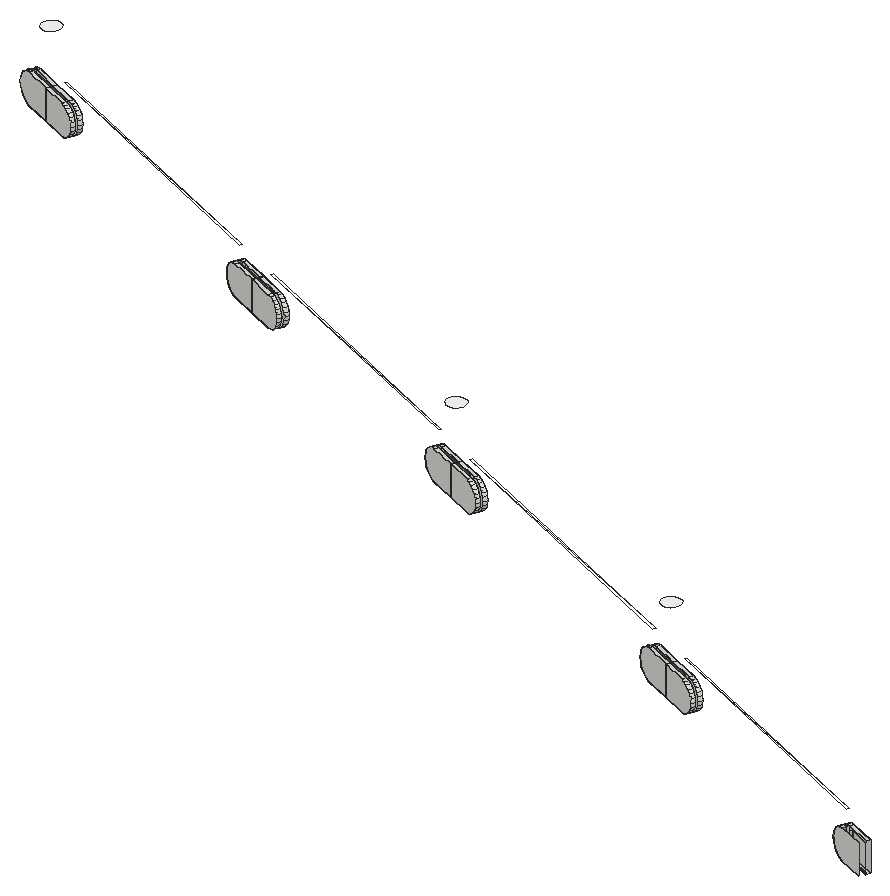
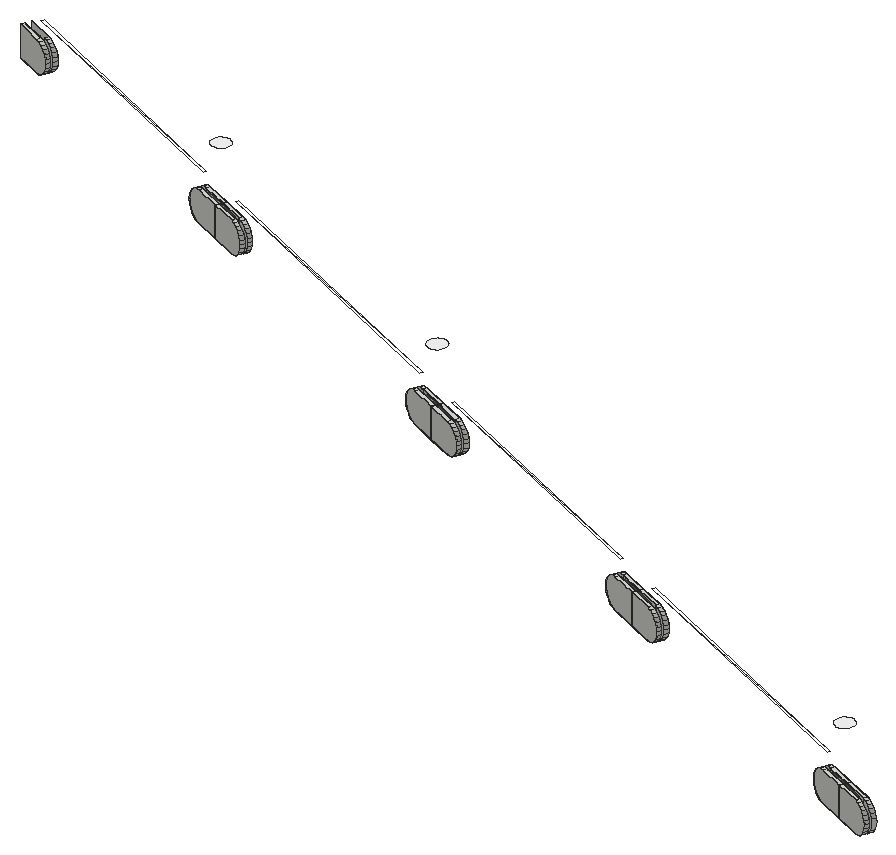
# SketchUp Ruby script. Lengths in inches.
U = 1.inch
M = Sketchup.active_model
def pt(a) = Geom::Point3d.new(a.map { |v| v * U })
def face(e, loops, mat)
  f = e.add_face(loops[0].map { |a| pt(a) })
  loops[1..].each { |l| e.add_face(l.map { |a| pt(a) }).erase! }
  f.material = f.back_material = mat if mat
  f
end
# faces: each face lists its corners as indices into pts; further lists are holes
def faces(e, pts, list, mat = nil) = list.each { |f| face(e, (f[0].is_a?(Array) ? f : [f]).map { |l| l.map { |i| pts[i] } }, mat) }
# xy, xz, yz: faces in a plane at the given z, y or x. An outline is a flat list of corners, or four numbers for a rectangle; further outlines are holes
def ring(l) = l.size == 4 ? [[l[0], l[1]], [l[2], l[1]], [l[2], l[3]], [l[0], l[3]]] : l.each_slice(2).to_a
def flat(e, list, mat, &to3) = list.each { |f| face(e, (f[0].is_a?(Array) ? f : [f]).map { |l| ring(l).map { |u, v| to3.(u, v) } }, mat) }
def xy(e, z, list, mat = nil) = flat(e, list, mat) { |x, y| [x, y, z] }
def xz(e, y, list, mat = nil) = flat(e, list, mat) { |x, z| [x, y, z] }
def yz(e, x, list, mat = nil) = flat(e, list, mat) { |y, z| [x, y, z] }
def lines(e, pts, list) = list.each { |a, b| e.add_line(pt(pts[a]), pt(pts[b])) }
# prism: a flat outline (further loops are holes) pulled along v
def prism(e, loops, v, mat = nil)
  f = face(e, loops, mat); d = Geom::Vector3d.new(v.map { |x| x * U })
  f.pushpull(f.normal.samedirection?(d) ? d.length : -d.length)
end
def box(e, o, s, mat = nil) = prism(e, [[o, [o[0] + s[0], o[1], o[2]], [o[0] + s[0], o[1] + s[1], o[2]], [o[0], o[1] + s[1], o[2]]]], [0, 0, s[2]], mat)
def at(x, y, z, deg = 0) = Geom::Transformation.translation(pt([x, y, z])) * Geom::Transformation.rotation(ORIGIN, Z_AXIS, deg.degrees)
def axes(o, x, y, z) = Geom::Transformation.new([*x, 0, *y, 0, *z, 0, *pt(o).to_a, 1])
def part(name) = M.definitions.add(name)
# library, detail: a bought-in or finely detailed component or shape, given as its bounding box
def library(name, o, s) = part(name).tap { |d| box(d.entities, o, s) }
def detail(e, o, s) = box(e.add_group.entities, o, s)
def put(e, d, t, mat = nil) = e.add_instance(d, t).tap { |i| i.material = mat if mat }
def group(e, t, mat = nil) = e.add_group.tap { |g| g.transformation = t; g.material = mat if mat }.entities
root = M.entities
M.materials.add("Glass_Safety_01").color = [204, 235, 244]
M.materials["Glass_Safety_01"].alpha = 0.1
M.materials.add("[Color_000]").color = [255, 255, 255]
xy(root,351.28,[[937.98,1050.01,936.18,1050.79,936.29,1051.04,938.09,1050.26],[918.36,1058.03,916.56,1058.82,916.67,1059.07,918.32,1058.35,918.47,1058.29],[918.55,1058.47,918.4,1058.53,916.75,1059.25,916.86,1059.51,918.66,1058.72],[916.56,1058.82,914.75,1059.61,914.86,1059.86,916.67,1059.07],[916.75,1059.25,914.94,1060.04,915.05,1060.29,916.86,1059.51],
  [894.73,1068.32,892.93,1069.11,893.04,1069.36,894.71,1068.64,894.84,1068.58],[894.92,1068.76,894.79,1068.82,893.12,1069.54,893.23,1069.8,895.03,1069.01],[892.93,1069.11,891.125,1069.9,891.24,1070.15,893.04,1069.36],[893.12,1069.54,891.3125,1070.33,891.42,1070.58,893.23,1069.8],[872.89,1077.84,871.09,1078.625,871.2,1078.88,872.85,1078.16,873,1078.09],
  [873.08,1078.27,872.93,1078.34,871.27,1079.06,871.38,1079.31,873.19,1078.52],[871.09,1078.625,869.28,1079.41,869.39,1079.66,871.2,1078.88],[871.27,1079.06,869.47,1079.84,869.58,1080.1,871.38,1079.31],[850.22,1087.71,848.42,1088.5,848.53,1088.75,850.19,1088.03,850.33,1087.96],[850.41,1088.14,850.27,1088.21,848.61,1088.93,848.72,1089.18,850.52,1088.4],
  [848.42,1088.5,846.62,1089.28,846.73,1089.54,848.53,1088.75],[848.61,1088.93,846.8,1089.72,846.91,1089.97,848.72,1089.18]])
xy(root,351.36,[[918.11,1058.44,916.67,1059.07,916.75,1059.25,918.19,1058.625],[916.67,1059.07,915.23,1059.7,915.3,1059.88,916.75,1059.25],[894.48,1068.73,893.04,1069.36,893.12,1069.54,894.5625,1068.92],[893.04,1069.36,891.6,1069.99,891.67,1070.17,893.12,1069.54],[872.64,1078.25,871.2,1078.88,871.27,1079.06,872.72,1078.43],
  [871.2,1078.88,869.75,1079.51,869.83,1079.6875,871.27,1079.06],[849.97,1088.12,848.53,1088.75,848.61,1088.93,850.05,1088.3],[848.53,1088.75,847.09,1089.38,847.16,1089.56,848.61,1088.93]],"Glass_Safety_01")
xy(root,353.33,[[918.11,1058.44,918.19,1058.625,916.75,1059.25,916.67,1059.07],[916.67,1059.07,916.75,1059.25,915.3,1059.88,915.23,1059.7],[894.48,1068.73,894.5625,1068.92,893.12,1069.54,893.04,1069.36],[893.04,1069.36,893.12,1069.54,891.67,1070.17,891.6,1069.99],[872.64,1078.25,872.72,1078.43,871.27,1079.06,871.2,1078.88],
  [871.2,1078.88,871.27,1079.06,869.83,1079.6875,869.75,1079.51],[849.97,1088.12,850.05,1088.3,848.61,1088.93,848.53,1088.75],[848.53,1088.75,848.61,1088.93,847.16,1089.56,847.09,1089.38]],"Glass_Safety_01")
xy(root,353.41,[[937.98,1050.01,938.09,1050.26,936.29,1051.04,936.18,1050.79],[918.36,1058.03,918.47,1058.29,918.32,1058.35,916.67,1059.07,916.56,1058.82],[918.55,1058.47,918.66,1058.72,916.86,1059.51,916.75,1059.25,918.4,1058.53],[916.56,1058.82,916.67,1059.07,914.86,1059.86,914.75,1059.61],[916.75,1059.25,916.86,1059.51,915.05,1060.29,914.94,1060.04],
  [894.73,1068.32,894.84,1068.58,894.71,1068.64,893.04,1069.36,892.93,1069.11],[894.92,1068.76,895.03,1069.01,893.23,1069.8,893.12,1069.54,894.79,1068.82],[892.93,1069.11,893.04,1069.36,891.24,1070.15,891.125,1069.9],[893.12,1069.54,893.23,1069.8,891.42,1070.58,891.3125,1070.33],[872.89,1077.84,873,1078.09,872.85,1078.16,871.2,1078.88,871.09,1078.625],
  [873.08,1078.27,873.19,1078.52,871.38,1079.31,871.27,1079.06,872.93,1078.34],[871.09,1078.625,871.2,1078.88,869.39,1079.66,869.28,1079.41],[871.27,1079.06,871.38,1079.31,869.58,1080.1,869.47,1079.84],[850.22,1087.71,850.33,1087.96,850.19,1088.03,848.53,1088.75,848.42,1088.5],[850.41,1088.14,850.52,1088.4,848.72,1089.18,848.61,1088.93,850.27,1088.21],
  [848.42,1088.5,848.53,1088.75,846.73,1089.54,846.62,1089.28],[848.61,1088.93,848.72,1089.18,846.91,1089.97,846.8,1089.72]])
xy(root,354.51,[[936.1,1050.61,936.18,1050.79,918.32,1058.35],[936.18,1050.79,918.4,1058.53,918.32,1058.35],[914.86,1059.86,914.94,1060.04,894.71,1068.64],[914.94,1060.04,894.79,1068.82,894.71,1068.64],[891.24,1070.15,891.3125,1070.33,872.85,1078.16],
  [891.3125,1070.33,872.93,1078.34,872.85,1078.16],[869.39,1079.66,869.47,1079.84,850.19,1088.03],[869.47,1079.84,850.27,1088.21,850.19,1088.03]],"Glass_Safety_01")
xy(root,357.27,[[916.75,1058.53,916.91,1058.57,917.0625,1058.64,917.18,1058.75,917.27,1058.89,917.33,1059.04,917.34,1059.21,917.3,1059.37,917.23,1059.52,917.12,1059.64,916.98,1059.73,916.83,1059.78,916.66,1059.79,916.5,1059.76,916.36,1059.68,916.23,1059.58,916.14,1059.4375,916.09,1059.28,916.08,1059.12,916.11,1058.96,916.1875,1058.81,916.3,1058.6875,916.43,1058.6,916.59,1058.54],[893.125,1068.83,893.29,1068.86,893.43,1068.93,893.56,1069.04,893.65,1069.18,893.7,1069.33,893.71,1069.5,893.67,1069.66,893.6,1069.81,893.49,1069.93,893.35,1070.02,893.2,1070.07,893.03,1070.08,892.875,1070.05,892.73,1069.98,892.6,1069.87,892.51,1069.73,892.46,1069.57,892.45,1069.41,892.48,1069.25,892.56,1069.1,892.67,1068.98,892.8,1068.89,892.96,1068.84],[848.61,1088.21,848.78,1088.24,848.92,1088.32,849.05,1088.43,849.14,1088.5625,849.1875,1088.72,849.2,1088.88,849.16,1089.05,849.09,1089.19,848.98,1089.32,848.84,1089.41,848.6875,1089.46,848.52,1089.47,848.36,1089.43,848.22,1089.36,848.09,1089.25,848,1089.11,847.95,1088.96,847.94,1088.79,847.97,1088.63,848.05,1088.49,848.16,1088.36,848.29,1088.27,848.45,1088.22]],"[Color_000]")
p = [[937.79,1049.57,353.41],[935.99,1050.36,353.41],[935.74,1050.47,353.37],[935.5,1050.57,353.27],[935.3,1050.66,353.1],[935.14,1050.73,352.88],
  [935.05,1050.77,352.62],[935.01,1050.78,352.35],[935.05,1050.77,352.07],[935.14,1050.73,351.8125],[935.3,1050.66,351.59],[935.5,1050.57,351.43],
  [935.74,1050.47,351.32],[935.99,1050.36,351.28],[937.79,1049.57,351.28],[937.98,1050.01,353.41],[936.18,1050.79,353.41],[936.18,1050.79,351.28],
  [937.98,1050.01,351.28],[937.98,1050.01,351.36],[936.54,1050.63,351.36],[936.54,1050.63,353.33],[937.98,1050.01,353.33],[936.29,1051.04,353.41],
  [938.09,1050.26,353.41],[938.09,1050.26,351.28],[936.29,1051.04,351.28],[936.03,1051.15,351.32],[935.8,1051.26,351.43],[935.6,1051.34,351.59],
  [935.44,1051.41,351.8125],[935.34,1051.45,352.07],[935.3125,1051.47,352.35],[935.34,1051.45,352.62],[935.44,1051.41,352.88],[935.6,1051.34,353.1],
  [935.8,1051.26,353.27],[936.03,1051.15,353.37],[935.85,1050.72,351.32],[936.1,1050.61,351.28],[935.61,1050.82,351.43],[936.1,1050.61,353.41],
  [935.85,1050.72,353.37],[935.61,1050.82,353.27],[935.41,1050.91,353.1],[935.25,1050.98,352.88],[935.16,1051.02,352.62],[935.12,1051.04,352.35],
  [935.16,1051.02,352.07],[935.25,1050.98,351.8125],[935.41,1050.91,351.59],[935.92,1050.9,351.32],[935.6875,1051,351.43],[935.49,1051.09,351.59],
  [935.33,1051.16,351.8125],[935.23,1051.2,352.07],[935.2,1051.22,352.35],[935.23,1051.2,352.62],[935.33,1051.16,352.88],[935.49,1051.09,353.1],
  [935.6875,1051,353.27],[935.92,1050.9,353.37],[918.36,1058.03,353.41],[916.56,1058.82,353.41],[916.56,1058.82,351.28],[918.36,1058.03,351.28],
  [918.62,1057.92,351.32],[918.85,1057.82,351.43],[919.05,1057.73,351.59],[919.21,1057.67,351.8125],[919.3,1057.625,352.07],[919.34,1057.61,352.35],
  [919.3,1057.625,352.62],[919.21,1057.67,352.88],[919.05,1057.73,353.1],[918.85,1057.82,353.27],[918.62,1057.92,353.37],[918.73,1058.18,351.32],
  [918.96,1058.07,351.43],[918.47,1058.29,351.28],[918.32,1058.35,351.28],[918.32,1058.35,353.41],[918.47,1058.29,353.41],[918.73,1058.18,353.37],
  [918.96,1058.07,353.27],[919.16,1057.99,353.1],[919.32,1057.92,352.88],[919.42,1057.875,352.62],[919.45,1057.86,352.35],[919.42,1057.875,352.07],
  [919.32,1057.92,351.8125],[919.16,1057.99,351.59],[918.55,1058.47,353.41],[918.4,1058.53,353.41],[918.4,1058.53,351.28],[918.55,1058.47,351.28],
  [918.8,1058.36,351.32],[919.04,1058.25,351.43],[919.24,1058.17,351.59],[919.4,1058.1,351.8125],[919.49,1058.06,352.07],[919.53,1058.04,352.35],
  [919.49,1058.06,352.62],[919.4,1058.1,352.88],[919.24,1058.17,353.1],[919.04,1058.25,353.27],[918.8,1058.36,353.37],[916.86,1059.51,353.41],
  [918.66,1058.72,353.41],[918.91,1058.61,353.37],[919.15,1058.51,353.27],[919.35,1058.42,353.1],[919.51,1058.35,352.88],[919.6,1058.31,352.62],
  [919.64,1058.3,352.35],[919.6,1058.31,352.07],[919.51,1058.35,351.8125],[919.35,1058.42,351.59],[919.15,1058.51,351.43],[918.91,1058.61,351.32],
  [918.66,1058.72,351.28],[916.86,1059.51,351.28],[916.67,1059.07,353.41],[916.67,1059.07,351.28],[916.67,1059.07,351.36],[918.11,1058.44,351.36],
  [918.11,1058.44,353.33],[916.67,1059.07,353.33],[916.75,1059.25,351.28],[916.75,1059.25,353.41],[916.75,1059.25,353.33],[918.19,1058.625,353.33],
  [918.19,1058.625,351.36],[916.75,1059.25,351.36],[914.75,1059.61,353.41],[914.5,1059.72,353.37],[914.27,1059.82,353.27],[914.06,1059.91,353.1],
  [913.91,1059.97,352.88],[913.8125,1060.02,352.62],[913.78,1060.03,352.35],[913.8125,1060.02,352.07],[913.91,1059.97,351.8125],[914.06,1059.91,351.59],
  [914.27,1059.82,351.43],[914.5,1059.72,351.32],[914.75,1059.61,351.28],[914.86,1059.86,351.28],[914.86,1059.86,353.41],[915.23,1059.7,353.33],
  [915.23,1059.7,351.36],[914.94,1060.04,353.41],[914.94,1060.04,351.28],[915.3,1059.88,351.36],[915.3,1059.88,353.33],[915.05,1060.29,353.41],
  [915.05,1060.29,351.28],[914.8,1060.4,351.32],[914.57,1060.5,351.43],[914.36,1060.59,351.59],[914.21,1060.66,351.8125],[914.11,1060.7,352.07],
  [914.08,1060.72,352.35],[914.11,1060.7,352.62],[914.21,1060.66,352.88],[914.36,1060.59,353.1],[914.57,1060.5,353.27],[914.8,1060.4,353.37],
  [914.61,1059.97,351.32],[914.375,1060.07,351.43],[914.61,1059.97,353.37],[914.375,1060.07,353.27],[914.17,1060.16,353.1],[914.02,1060.23,352.88],
  [913.92,1060.27,352.62],[913.89,1060.28,352.35],[913.92,1060.27,352.07],[914.02,1060.23,351.8125],[914.17,1060.16,351.59],[914.69,1060.15,351.32],
  [914.46,1060.25,351.43],[914.25,1060.34,351.59],[914.1,1060.41,351.8125],[914,1060.45,352.07],[913.97,1060.46,352.35],[914,1060.45,352.62],
  [914.1,1060.41,352.88],[914.25,1060.34,353.1],[914.46,1060.25,353.27],[914.69,1060.15,353.37],[894.73,1068.32,353.41],[892.93,1069.11,353.41],
  [892.93,1069.11,351.28],[894.73,1068.32,351.28],[894.99,1068.22,351.32],[895.22,1068.11,351.43],[895.42,1068.02,351.59],[895.58,1067.96,351.8125],
  [895.68,1067.91,352.07],[895.71,1067.9,352.35],[895.68,1067.91,352.62],[895.58,1067.96,352.88],[895.42,1068.02,353.1],[895.22,1068.11,353.27],
  [894.99,1068.22,353.37],[895.1,1068.47,351.32],[895.33,1068.37,351.43],[894.84,1068.58,351.28],[894.71,1068.64,351.28],[894.71,1068.64,353.41],
  [894.84,1068.58,353.41],[895.1,1068.47,353.37],[895.33,1068.37,353.27],[895.53,1068.28,353.1],[895.6875,1068.21,352.88],[895.79,1068.17,352.62],
  [895.82,1068.15,352.35],[895.79,1068.17,352.07],[895.6875,1068.21,351.8125],[895.53,1068.28,351.59],[894.92,1068.76,353.41],[894.79,1068.82,353.41],
  [894.79,1068.82,351.28],[894.92,1068.76,351.28],[895.18,1068.65,351.32],[895.41,1068.55,351.43],[895.61,1068.46,351.59],[895.77,1068.39,351.8125],
  [895.86,1068.35,352.07],[895.9,1068.33,352.35],[895.86,1068.35,352.62],[895.77,1068.39,352.88],[895.61,1068.46,353.1],[895.41,1068.55,353.27],
  [895.18,1068.65,353.37],[895.29,1068.9,351.32],[895.52,1068.8,351.43],[893.04,1069.36,353.41],[893.04,1069.36,351.28],[893.04,1069.36,351.36],
  [894.48,1068.73,351.36],[894.48,1068.73,353.33],[893.04,1069.36,353.33],[893.23,1069.8,353.41],[895.03,1069.01,353.41],[895.29,1068.9,353.37],
  [895.52,1068.8,353.27],[895.72,1068.71,353.1],[895.88,1068.64,352.88],[895.97,1068.6,352.62],[896.01,1068.59,352.35],[895.97,1068.6,352.07],
  [895.88,1068.64,351.8125],[895.72,1068.71,351.59],[895.03,1069.01,351.28],[893.23,1069.8,351.28],[893.12,1069.54,351.28],[893.12,1069.54,353.41],
  [893.12,1069.54,353.33],[894.5625,1068.92,353.33],[894.5625,1068.92,351.36],[893.12,1069.54,351.36],[891.125,1069.9,353.41],[890.87,1070.01,353.37],
  [890.64,1070.11,353.27],[890.4375,1070.2,353.1],[890.28,1070.26,352.88],[890.18,1070.31,352.62],[890.15,1070.32,352.35],[890.18,1070.31,352.07],
  [890.28,1070.26,351.8125],[890.4375,1070.2,351.59],[890.64,1070.11,351.43],[890.87,1070.01,351.32],[891.125,1069.9,351.28],[891.24,1070.15,351.28],
  [891.24,1070.15,353.41],[891.6,1069.99,353.33],[891.6,1069.99,351.36],[891.3125,1070.33,353.41],[891.3125,1070.33,351.28],[891.67,1070.17,351.36],
  [891.67,1070.17,353.33],[891.42,1070.58,353.41],[891.42,1070.58,351.28],[891.17,1070.69,351.32],[890.9375,1070.79,351.43],[890.73,1070.88,351.59],
  [890.58,1070.95,351.8125],[890.48,1070.99,352.07],[890.45,1071.01,352.35],[890.48,1070.99,352.62],[890.58,1070.95,352.88],[890.73,1070.88,353.1],
  [890.9375,1070.79,353.27],[891.17,1070.69,353.37],[890.98,1070.26,351.32],[890.75,1070.36,351.43],[890.98,1070.26,353.37],[890.75,1070.36,353.27],
  [890.55,1070.45,353.1],[890.39,1070.52,352.88],[890.29,1070.56,352.62],[890.26,1070.57,352.35],[890.29,1070.56,352.07],[890.39,1070.52,351.8125],
  [890.55,1070.45,351.59],[891.0625,1070.44,351.32],[890.83,1070.54,351.43],[890.625,1070.63,351.59],[890.47,1070.7,351.8125],[890.37,1070.74,352.07],
  [890.34,1070.75,352.35],[890.37,1070.74,352.62],[890.47,1070.7,352.88],[890.625,1070.63,353.1],[890.83,1070.54,353.27],[891.0625,1070.44,353.37],
  [872.89,1077.84,353.41],[871.09,1078.625,353.41],[871.09,1078.625,351.28],[872.89,1077.84,351.28],[873.14,1077.73,351.32],[873.38,1077.625,351.43],
  [873.58,1077.54,351.59],[873.73,1077.47,351.8125],[873.83,1077.43,352.07],[873.87,1077.41,352.35],[873.83,1077.43,352.62],[873.73,1077.47,352.88],
  [873.58,1077.54,353.1],[873.38,1077.625,353.27],[873.14,1077.73,353.37],[873.25,1077.98,351.32],[873.49,1077.88,351.43],[873,1078.09,351.28],
  [872.85,1078.16,351.28],[872.85,1078.16,353.41],[873,1078.09,353.41],[873.25,1077.98,353.37],[873.49,1077.88,353.27],[873.69,1077.79,353.1],
  [873.84,1077.72,352.88],[873.94,1077.68,352.62],[873.98,1077.67,352.35],[873.94,1077.68,352.07],[873.84,1077.72,351.8125],[873.69,1077.79,351.59],
  [873.08,1078.27,353.41],[872.93,1078.34,353.41],[872.93,1078.34,351.28],[873.08,1078.27,351.28],[873.33,1078.16,351.32],[873.57,1078.06,351.43],
  [873.77,1077.97,351.59],[873.92,1077.9,351.8125],[874.02,1077.86,352.07],[874.05,1077.85,352.35],[874.02,1077.86,352.62],[873.92,1077.9,352.88],
  [873.77,1077.97,353.1],[873.57,1078.06,353.27],[873.33,1078.16,353.37],[871.38,1079.31,353.41],[873.19,1078.52,353.41],[873.44,1078.41,353.37],
  [873.68,1078.3125,353.27],[873.88,1078.22,353.1],[874.03,1078.16,352.88],[874.13,1078.11,352.62],[874.16,1078.1,352.35],[874.13,1078.11,352.07],
  [874.03,1078.16,351.8125],[873.88,1078.22,351.59],[873.68,1078.3125,351.43],[873.44,1078.41,351.32],[873.19,1078.52,351.28],[871.38,1079.31,351.28],
  [871.2,1078.88,353.41],[871.2,1078.88,351.28],[871.2,1078.88,351.36],[872.64,1078.25,351.36],[872.64,1078.25,353.33],[871.2,1078.88,353.33],
  [871.27,1079.06,351.28],[871.27,1079.06,353.41],[871.27,1079.06,353.33],[872.72,1078.43,353.33],[872.72,1078.43,351.36],[871.27,1079.06,351.36],
  [869.28,1079.41,353.41],[869.03,1079.52,353.37],[868.79,1079.62,353.27],[868.59,1079.71,353.1],[868.4375,1079.78,352.88],[868.34,1079.82,352.62],
  [868.31,1079.84,352.35],[868.34,1079.82,352.07],[868.4375,1079.78,351.8125],[868.59,1079.71,351.59],[868.79,1079.62,351.43],[869.03,1079.52,351.32],
  [869.28,1079.41,351.28],[869.39,1079.66,351.28],[869.39,1079.66,353.41],[869.75,1079.51,353.33],[869.75,1079.51,351.36],[869.47,1079.84,353.41],
  [869.47,1079.84,351.28],[869.83,1079.6875,351.36],[869.83,1079.6875,353.33],[869.58,1080.1,353.41],[869.58,1080.1,351.28],[869.33,1080.21,351.32],
  [869.09,1080.31,351.43],[868.89,1080.4,351.59],[868.74,1080.46,351.8125],[868.64,1080.51,352.07],[868.61,1080.52,352.35],[868.64,1080.51,352.62],
  [868.74,1080.46,352.88],[868.89,1080.4,353.1],[869.09,1080.31,353.27],[869.33,1080.21,353.37],[869.14,1079.77,351.32],[868.9,1079.875,351.43],
  [869.14,1079.77,353.37],[868.9,1079.875,353.27],[868.7,1079.96,353.1],[868.55,1080.03,352.88],[868.45,1080.07,352.62],[868.42,1080.09,352.35],
  [868.45,1080.07,352.07],[868.55,1080.03,351.8125],[868.7,1079.96,351.59],[869.22,1079.95,351.32],[868.98,1080.06,351.43],[868.78,1080.14,351.59],
  [868.625,1080.21,351.8125],[868.53,1080.25,352.07],[868.5,1080.27,352.35],[868.53,1080.25,352.62],[868.625,1080.21,352.88],[868.78,1080.14,353.1],
  [868.98,1080.06,353.27],[869.22,1079.95,353.37],[850.22,1087.71,353.41],[848.42,1088.5,353.41],[848.42,1088.5,351.28],[850.22,1087.71,351.28],
  [850.48,1087.6,351.32],[850.71,1087.5,351.43],[850.91,1087.41,351.59],[851.07,1087.34,351.8125],[851.17,1087.3,352.07],[851.2,1087.29,352.35],
  [851.17,1087.3,352.62],[851.07,1087.34,352.88],[850.91,1087.41,353.1],[850.71,1087.5,353.27],[850.48,1087.6,353.37],[850.33,1087.96,351.28],
  [850.19,1088.03,351.28],[850.19,1088.03,353.41],[850.33,1087.96,353.41],[850.59,1087.85,353.37],[850.82,1087.75,353.27],[851.02,1087.66,353.1],
  [851.18,1087.6,352.88],[851.28,1087.55,352.62],[851.31,1087.54,352.35],[851.28,1087.55,352.07],[851.18,1087.6,351.8125],[851.02,1087.66,351.59],
  [850.82,1087.75,351.43],[850.59,1087.85,351.32],[850.41,1088.14,353.41],[850.27,1088.21,353.41],[850.27,1088.21,351.28],[850.41,1088.14,351.28],
  [850.67,1088.03,351.32],[850.9,1087.93,351.43],[851.1,1087.84,351.59],[851.26,1087.78,351.8125],[851.35,1087.73,352.07],[851.39,1087.72,352.35],
  [851.35,1087.73,352.62],[851.26,1087.78,352.88],[851.1,1087.84,353.1],[850.9,1087.93,353.27],[850.67,1088.03,353.37],[850.78,1088.29,351.32],
  [851.01,1088.18,351.43],[848.53,1088.75,353.41],[848.53,1088.75,351.28],[848.53,1088.75,351.36],[849.97,1088.12,351.36],[849.97,1088.12,353.33],
  [848.53,1088.75,353.33],[848.72,1089.18,353.41],[850.52,1088.4,353.41],[850.78,1088.29,353.37],[851.01,1088.18,353.27],[851.21,1088.1,353.1],
  [851.37,1088.03,352.88],[851.46,1087.99,352.62],[851.5,1087.97,352.35],[851.46,1087.99,352.07],[851.37,1088.03,351.8125],[851.21,1088.1,351.59],
  [850.52,1088.4,351.28],[848.72,1089.18,351.28],[848.61,1088.93,351.28],[848.61,1088.93,353.41],[848.61,1088.93,353.33],[850.05,1088.3,353.33],
  [850.05,1088.3,351.36],[848.61,1088.93,351.36],[846.62,1089.28,353.41],[846.36,1089.39,353.37],[846.13,1089.49,353.27],[845.93,1089.58,353.1],
  [845.77,1089.65,352.88],[845.67,1089.69,352.62],[845.64,1089.71,352.35],[845.67,1089.69,352.07],[845.77,1089.65,351.8125],[845.93,1089.58,351.59],
  [846.13,1089.49,351.43],[846.36,1089.39,351.32],[846.62,1089.28,351.28],[846.73,1089.54,351.28],[846.73,1089.54,353.41],[847.09,1089.38,353.33],
  [847.09,1089.38,351.36],[846.8,1089.72,353.41],[846.8,1089.72,351.28],[847.16,1089.56,351.36],[847.16,1089.56,353.33],[846.91,1089.97,353.41],
  [846.91,1089.97,351.28],[846.66,1090.08,351.32],[846.43,1090.18,351.43],[846.22,1090.27,351.59],[846.07,1090.34,351.8125],[845.97,1090.38,352.07],
  [845.9375,1090.39,352.35],[845.97,1090.38,352.62],[846.07,1090.34,352.88],[846.22,1090.27,353.1],[846.43,1090.18,353.27],[846.66,1090.08,353.37],
  [846.47,1089.64,351.32],[846.24,1089.75,351.43],[846.47,1089.64,353.37],[846.24,1089.75,353.27],[846.04,1089.84,353.1],[845.88,1089.9,352.88],
  [845.78,1089.95,352.62],[845.75,1089.96,352.35],[845.78,1089.95,352.07],[845.88,1089.9,351.8125],[846.04,1089.84,351.59],[846.55,1089.83,351.32],
  [846.32,1089.93,351.43],[846.11,1090.02,351.59],[845.96,1090.08,351.8125],[845.86,1090.125,352.07],[845.83,1090.14,352.35],[845.86,1090.125,352.62],
  [845.96,1090.08,352.88],[846.11,1090.02,353.1],[846.32,1089.93,353.27],[846.55,1089.83,353.37],[936.46,1050.45,351.36],[936.46,1050.45,353.33]]
faces(root,p,[[0,1,2,3,4,5,6,7,8,9,10,11,12,13,14],[15,16,17,18,19,20,21,22],[23,24,25,26,27,28,29,30,31,32,33,34,35,36,37],[38,39,13,12],[40,38,12,11],[17,51,27,26],[51,52,28,27],[62,63,64,65,66,67,68,69,70,71,72,73,74,75,76],
  [77,78,67,66],[79,80,81,82,83,84,85,86,87,88,89,90,91,78,77],[79,77,66,65],[92,93,94,95,96,97,98,99,100,101,102,103,104,105,106],[107,108,109,110,111,112,113,114,115,116,117,118,119,120,121],[97,96,119,118],[122,81,80,123,124,125,126,127],[96,95,120,119],
  [128,94,93,129,130,131,132,133],[63,134,135,136,137,138,139,140,141,142,143,144,145,146,64],[124,123,64,63,122,127],[123,147,148,122,127,149,150,124],[129,151,152,128,133,153,154,130],[128,133,130,129,107,121],[155,107,121,156,157,158,159,160,161,162,163,164,165,166,167],[168,147,146,145],
  [169,168,145,144],[152,179,157,156],[179,180,158,157],[190,191,192,193,194,195,196,197,198,199,200,201,202,203,204],[205,206,195,194],[207,208,209,210,211,212,213,214,215,216,217,218,219,206,205],[207,205,194,193],[220,221,222,223,224,225,226,227,228,229,230,231,232,233,234],
  [225,224,235,236],[237,209,208,238,239,240,241,242],[243,244,245,246,247,248,249,250,251,252,253,236,235,254,255],[224,223,254,235],[256,222,221,257,258,259,260,261],[191,262,263,264,265,266,267,268,269,270,271,272,273,274,192],[239,238,192,191,237,242],[238,275,276,237,242,277,278,239],
  [257,279,280,256,261,281,282,258],[256,261,258,257,243,255],[283,243,255,284,285,286,287,288,289,290,291,292,293,294,295],[296,275,274,273],[297,296,273,272],[280,307,285,284],[307,308,286,285],[318,319,320,321,322,323,324,325,326,327,328,329,330,331,332],
  [333,334,323,322],[335,336,337,338,339,340,341,342,343,344,345,346,347,334,333],[335,333,322,321],[348,349,350,351,352,353,354,355,356,357,358,359,360,361,362],[363,364,365,366,367,368,369,370,371,372,373,374,375,376,377],[353,352,375,374],[378,337,336,379,380,381,382,383],[352,351,376,375],
  [384,350,349,385,386,387,388,389],[319,390,391,392,393,394,395,396,397,398,399,400,401,402,320],[380,379,320,319,378,383],[379,403,404,378,383,405,406,380],[385,407,408,384,389,409,410,386],[384,389,386,385,363,377],[411,363,377,412,413,414,415,416,417,418,419,420,421,422,423],[424,403,402,401],
  [425,424,401,400],[408,435,413,412],[435,436,414,413],[446,447,448,449,450,451,452,453,454,455,456,457,458,459,460],[461,462,463,464,465,466,467,468,469,470,471,472,473,474,475],[475,474,451,450],[461,475,450,449],[476,477,478,479,480,481,482,483,484,485,486,487,488,489,490],
  [481,480,491,492],[493,463,462,494,495,496,497,498],[499,500,501,502,503,504,505,506,507,508,509,492,491,510,511],[480,479,510,491],[512,478,477,513,514,515,516,517],[447,518,519,520,521,522,523,524,525,526,527,528,529,530,448],[495,494,448,447,493,498],[494,531,532,493,498,533,534,495],
  [513,535,536,512,517,537,538,514],[512,517,514,513,499,511],[539,499,511,540,541,542,543,544,545,546,547,548,549,550,551],[552,531,530,529],[553,552,529,528],[536,563,541,540],[563,564,542,541],[50,40,11,10],
  [52,53,29,28],[78,91,68,67],[98,97,118,117],[178,169,144,143],[180,181,159,158],[206,219,196,195],[226,225,236,253],[306,297,272,271],
  [308,309,287,286],[334,347,324,323],[354,353,374,373],[434,425,400,399],[436,437,415,414],[474,473,452,451],[482,481,492,509],[562,553,528,527],
  [564,565,543,542],[49,50,10,9],[53,54,30,29],[91,90,69,68],[99,98,117,116],[177,178,143,142],[181,182,160,159],[219,218,197,196],
  [227,226,253,252],[305,306,271,270],[309,310,288,287],[347,346,325,324],[355,354,373,372],[433,434,399,398],[437,438,416,415],[473,472,453,452],
  [483,482,509,508],[561,562,527,526],[565,566,544,543],[48,49,9,8],[54,55,31,30],[90,89,70,69],[100,99,116,115],[176,177,142,141],
  [182,183,161,160],[218,217,198,197],[228,227,252,251],[304,305,270,269],[310,311,289,288],[346,345,326,325],[356,355,372,371],[432,433,398,397],
  [438,439,417,416],[472,471,454,453],[484,483,508,507],[566,567,545,544],[47,48,8,7],[55,56,32,31],[89,88,71,70],[101,100,115,114],
  [175,176,141,140],[183,184,162,161],[217,216,199,198],[229,228,251,250],[303,304,269,268],[311,312,290,289],[345,344,327,326],[357,356,371,370],
  [431,432,397,396],[439,440,418,417],[471,470,455,454],[485,484,507,506],[567,568,546,545],[46,47,7,6],[56,57,33,32],[88,87,72,71],
  [102,101,114,113],[174,175,140,139],[184,185,163,162],[216,215,200,199],[230,229,250,249],[302,303,268,267],[312,313,291,290],[344,343,328,327],
  [358,357,370,369],[430,431,396,395],[440,441,419,418],[470,469,456,455],[486,485,506,505],[568,569,547,546],[45,46,6,5],[57,58,34,33],
  [87,86,73,72],[103,102,113,112],[173,174,139,138],[185,186,164,163],[215,214,201,200],[231,230,249,248],[301,302,267,266],[313,314,292,291],
  [343,342,329,328],[359,358,369,368],[429,430,395,394],[441,442,420,419],[469,468,457,456],[487,486,505,504],[557,558,523,522],[569,570,548,547],
  [44,45,5,4],[58,59,35,34],[86,85,74,73],[104,103,112,111],[172,173,138,137],[186,187,165,164],[214,213,202,201],[232,231,248,247],
  [300,301,266,265],[314,315,293,292],[342,341,330,329],[360,359,368,367],[428,429,394,393],[442,443,421,420],[468,467,458,457],[488,487,504,503],
  [556,557,522,521],[570,571,549,548],[43,44,4,3],[59,60,36,35],[85,84,75,74],[105,104,111,110],[171,172,137,136],[187,188,166,165],
  [213,212,203,202],[233,232,247,246],[299,300,265,264],[315,316,294,293],[341,340,331,330],[361,360,367,366],[427,428,393,392],[443,444,422,421],
  [467,466,459,458],[489,488,503,502],[555,556,521,520],[571,572,550,549],[42,43,3,2],[60,61,37,36],[84,83,76,75],[106,105,110,109],
  [170,171,136,135],[188,189,167,166],[212,211,204,203],[234,233,246,245],[298,299,264,263],[316,317,295,294],[340,339,332,331],[362,361,366,365],
  [426,427,392,391],[444,445,423,422],[466,465,460,459],[490,489,502,501],[554,555,520,519],[572,573,551,550],[41,42,2,1],[61,16,23,37],
  [83,82,62,76],[92,106,109,108],[148,170,135,134],[189,151,155,167],[211,210,190,204],[220,234,245,244],[276,298,263,262],[317,279,283,295],
  [339,338,318,332],[348,362,365,364],[404,426,391,390],[445,407,411,423],[465,464,446,460],[476,490,501,500],[532,554,519,518],[573,535,539,551]])
faces(root,p,[[39,41,42,43,44,45,46,47,48,49,50,40,38],[16,17,51,52,53,54,55,56,57,58,59,60,61],[147,148,170,171,172,173,174,175,176,177,178,169,168],[151,152,179,180,181,182,183,184,185,186,187,188,189],[275,276,298,299,300,301,302,303,304,305,306,297,296],[279,280,307,308,309,310,311,312,313,314,315,316,317],[403,404,426,427,428,429,430,431,432,433,434,425,424],[407,408,435,436,437,438,439,440,441,442,443,444,445],
  [531,532,554,555,556,557,558,559,560,561,562,553,552],[535,536,563,564,565,566,567,568,569,570,571,572,573],[22,21,20,19],[21,20,574,575],[127,126,125,124],[126,125,132,131],[131,130,133,132],[149,127,124,150],
  [127,130,133,124],[130,154,153,133],[154,153,150,149],[242,241,240,239],[241,240,260,259],[259,258,261,260],[277,242,239,278],[242,258,261,239],
  [258,282,281,261],[282,281,278,277],[383,382,381,380],[382,381,388,387],[387,386,389,388],[405,383,380,406],[383,386,389,380],[386,410,409,389],
  [410,409,406,405],[498,497,496,495],[497,496,516,515],[515,514,517,516],[533,498,495,534],[498,514,517,495],[514,538,537,517],[538,537,534,533]],"Glass_Safety_01")
